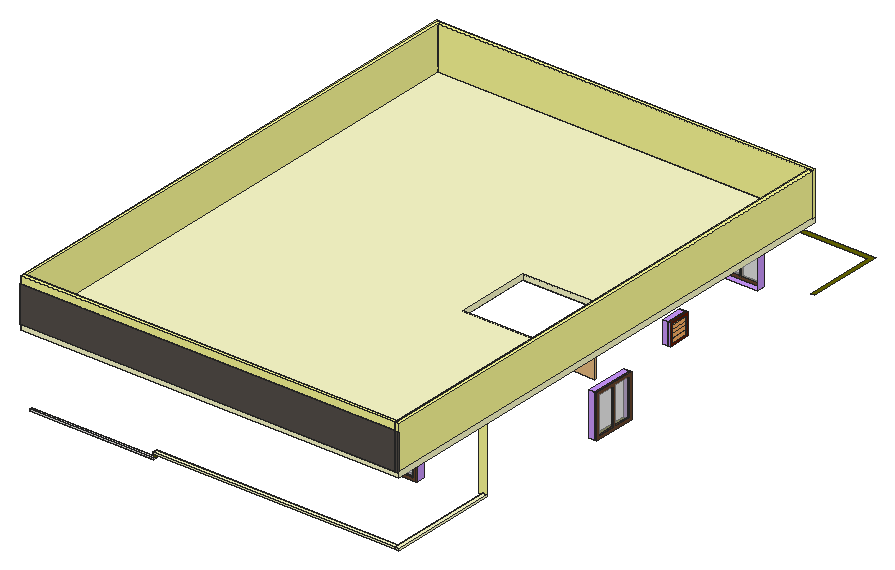
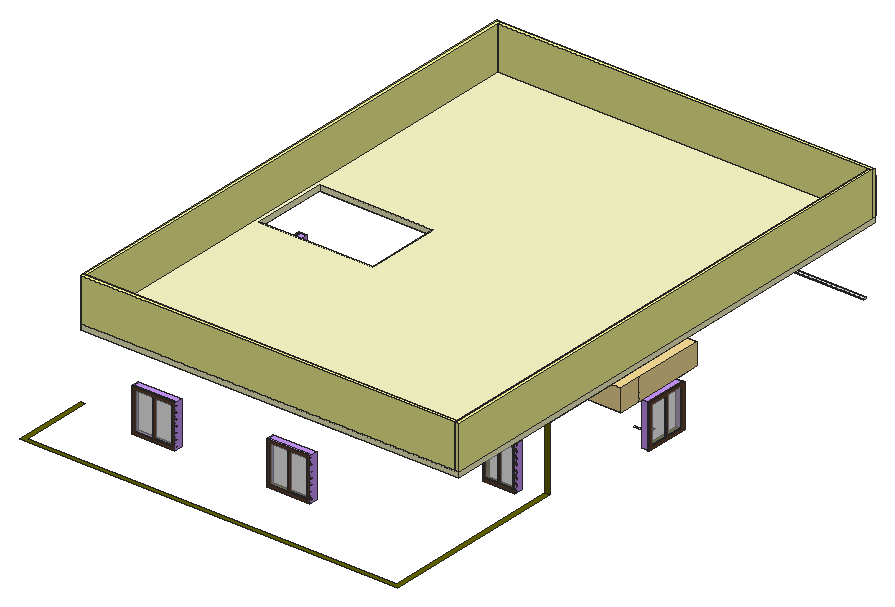
# SketchUp Ruby script. Lengths in inches.
U = 1.inch
M = Sketchup.active_model
def pt(a) = Geom::Point3d.new(a.map { |v| v * U })
def face(e, loops, mat)
  f = e.add_face(loops[0].map { |a| pt(a) })
  loops[1..].each { |l| e.add_face(l.map { |a| pt(a) }).erase! }
  f.material = f.back_material = mat if mat
  f
end
# faces: each face lists its corners as indices into pts; further lists are holes
def faces(e, pts, list, mat = nil) = list.each { |f| face(e, (f[0].is_a?(Array) ? f : [f]).map { |l| l.map { |i| pts[i] } }, mat) }
# xy, xz, yz: faces in a plane at the given z, y or x. An outline is a flat list of corners, or four numbers for a rectangle; further outlines are holes
def ring(l) = l.size == 4 ? [[l[0], l[1]], [l[2], l[1]], [l[2], l[3]], [l[0], l[3]]] : l.each_slice(2).to_a
def flat(e, list, mat, &to3) = list.each { |f| face(e, (f[0].is_a?(Array) ? f : [f]).map { |l| ring(l).map { |u, v| to3.(u, v) } }, mat) }
def xy(e, z, list, mat = nil) = flat(e, list, mat) { |x, y| [x, y, z] }
def xz(e, y, list, mat = nil) = flat(e, list, mat) { |x, z| [x, y, z] }
def yz(e, x, list, mat = nil) = flat(e, list, mat) { |y, z| [x, y, z] }
def lines(e, pts, list) = list.each { |a, b| e.add_line(pt(pts[a]), pt(pts[b])) }
# prism: a flat outline (further loops are holes) pulled along v
def prism(e, loops, v, mat = nil)
  f = face(e, loops, mat); d = Geom::Vector3d.new(v.map { |x| x * U })
  f.pushpull(f.normal.samedirection?(d) ? d.length : -d.length)
end
def box(e, o, s, mat = nil) = prism(e, [[o, [o[0] + s[0], o[1], o[2]], [o[0] + s[0], o[1] + s[1], o[2]], [o[0], o[1] + s[1], o[2]]]], [0, 0, s[2]], mat)
def at(x, y, z, deg = 0) = Geom::Transformation.translation(pt([x, y, z])) * Geom::Transformation.rotation(ORIGIN, Z_AXIS, deg.degrees)
def axes(o, x, y, z) = Geom::Transformation.new([*x, 0, *y, 0, *z, 0, *pt(o).to_a, 1])
def part(name) = M.definitions.add(name)
# library, detail: a bought-in or finely detailed component or shape, given as its bounding box
def library(name, o, s) = part(name).tap { |d| box(d.entities, o, s) }
def detail(e, o, s) = box(e.add_group.entities, o, s)
def put(e, d, t, mat = nil) = e.add_instance(d, t).tap { |i| i.material = mat if mat }
def group(e, t, mat = nil) = e.add_group.tap { |g| g.transformation = t; g.material = mat if mat }.entities
root = M.entities
M.materials.add("B08_Burnt_Sienna").color = [102, 25, 0]
M.materials.add("C03_Honey_Glow").color = [255, 178, 101]
M.materials.add("D02_Buttercup_Glow").color = [255, 229, 155]
M.materials.add("E01_Mint_Frost").color = [255, 255, 204]
M.materials.add("E02_Pale_Lime").color = [255, 255, 153]
M.materials.add("E08_Lime_Depth").color = [102, 102, 0]
M.materials.add("F06_Grassy_Shade").color = [102, 204, 0]
M.materials.add("G07_Jungle_Burst").color = [0, 153, 0]
M.materials.add("Glass_Mirror_01").color = [185, 185, 185]
M.materials["Glass_Mirror_01"].alpha = 0.91
M.materials.add("Glass_Mirror_2").color = [185, 185, 185]
M.materials["Glass_Mirror_2"].alpha = 0.8
M.materials.add("Glass_Mirror_3").color = [185, 185, 185]
M.materials["Glass_Mirror_3"].alpha = 0.65
M.materials.add("Glass_Mirror_4").color = [185, 185, 185]
M.materials["Glass_Mirror_4"].alpha = 0.68
M.materials.add("H06_Ocean_Depth").color = [0, 204, 204]
M.materials.add("H08_Emerald_Abyss").color = [0, 102, 102]
M.materials.add("I03_Bluebell_Mist").color = [101, 101, 255]
M.materials.add("I08_Inkstorm").color = [0, 0, 102]
M.materials.add("J02_Lavender_Veil").color = [204, 153, 255]
M.materials.add("J03_Orchid_Glow").color = [178, 101, 255]
M.materials.add("K02_Rosy_Glow").color = [255, 153, 255]
M.materials.add("M07_Charcoal_Gleam").color = [58, 58, 58]
M.materials.add("M09_Shadow_Night").color = [0, 0, 0]
M.materials.add("Metal_06_1K").color = [238, 236, 231]
M.materials.add("Roofing_01_1K").color = [84, 79, 73]
M.materials.add("Wood_Veneer_15_1K").color = [103, 69, 45]
c1 = part("Group\#57")
xy(c1.entities,0,[[0,-2,48,0]],"Wood_Veneer_15_1K")
xy(c1.entities,3,[[3,-2,23,0],[25,-2,45,0]],"Wood_Veneer_15_1K")
xy(c1.entities,45,[[3,-2,23,0],[25,-2,45,0]],"Wood_Veneer_15_1K")
xy(c1.entities,48,[[0,-2,48,0]],"Wood_Veneer_15_1K")
xz(c1.entities,-2,[[[0,0,48,48],[25,3,45,45],[3,3,23,45]]],"Wood_Veneer_15_1K")
xz(c1.entities,0,[[3,3,23,45],[25,3,45,45]],"Glass_Mirror_4")
xz(c1.entities,0,[[[0,0,48,48],[25,3,45,45],[3,3,23,45]]],"Wood_Veneer_15_1K")
yz(c1.entities,0,[[-2,0,0,48]],"Wood_Veneer_15_1K")
yz(c1.entities,3,[[-2,3,0,45]],"Wood_Veneer_15_1K")
yz(c1.entities,23,[[-2,3,0,45]],"Wood_Veneer_15_1K")
yz(c1.entities,25,[[-2,3,0,45]],"Wood_Veneer_15_1K")
yz(c1.entities,45,[[-2,3,0,45]],"Wood_Veneer_15_1K")
yz(c1.entities,48,[[-2,0,0,48]],"Wood_Veneer_15_1K")
c2 = library("Group\#24",[0,0,0],[4.375,4.375,0.1875])
c3 = part("Group\#8")
g1 = group(c3.entities,at(0.75,15.42,1.1875),"M07_Charcoal_Gleam")
prism(g1,[[[1.25,5.68,0],[1.25,0.93,0],[0.46,0.6,0],[0.3125,0.54,0],[0.18,0.44,0],[0.08,0.3125,0],[0.02,0.16,0],[0,0,0],[0,6.6875,0],[0.02,6.53,0],[0.08,6.375,0],[0.18,6.25,0],[0.3125,6.15,0],[0.46,6.08,0],[0.625,6.0625,0]]],[0,0,3.25])
g2 = group(c3.entities,at(0,11.83,0))
box(g2,[0,0,0],[2.8125,14.875,1.1875],"M07_Charcoal_Gleam")
g3 = group(c3.entities,at(2,0,4.4375))
xy(g3,0,[[-1,0,0,37.44]],"M07_Charcoal_Gleam")
xy(g3,21.9,[[-1,0,0,37.44]],"M07_Charcoal_Gleam")
xz(g3,0,[[-1,0,0,21.9]],"M07_Charcoal_Gleam")
xz(g3,37.44,[[-1,0,0,21.9]],"M07_Charcoal_Gleam")
yz(g3,-1,[[1.62,1.96,35.68,20.27]],"Glass_Mirror_01")
yz(g3,-1,[[[0,0,37.44,21.9],[1.62,1.96,35.68,20.27]]],"M07_Charcoal_Gleam")
yz(g3,0,[[[0,0,37.44,21.9],[1.62,1.96,35.68,20.27]]],"M07_Charcoal_Gleam")
p = [[0,35.68,20.27],[-1,35.68,20.27],[0,1.62,20.27],[-1,1.62,20.27],[0,35.68,1.96],[-1,35.68,1.96],
  [0,1.62,1.96],[-1,1.62,1.96]]
lines(g3,p,[[0,1],[2,3],[4,5],[6,7]])
c4 = part("Group\#56")
xy(c4.entities,0,[[0,0,2,48]],"Wood_Veneer_15_1K")
xy(c4.entities,3,[[0,3,2,23],[0,25,2,45]],"Wood_Veneer_15_1K")
xy(c4.entities,45.04,[[0,3,2,23],[0,25,2,45]],"Wood_Veneer_15_1K")
xy(c4.entities,48.04,[[0,0,2,48]],"Wood_Veneer_15_1K")
xz(c4.entities,0,[[0,0,2,48.04]],"Wood_Veneer_15_1K")
xz(c4.entities,3,[[0,3,2,23.02],[0,23.02,2,25.02],[0,25.02,2,45.04]],"Wood_Veneer_15_1K")
xz(c4.entities,23,[[0,3,2,23.02],[0,23.02,2,25.02],[0,25.02,2,45.04]],"Wood_Veneer_15_1K")
xz(c4.entities,25,[[0,3,2,23.02],[0,23.02,2,25.02],[0,25.02,2,45.04]],"Wood_Veneer_15_1K")
xz(c4.entities,45,[[0,3,2,23.02],[0,23.02,2,25.02],[0,25.02,2,45.04]],"Wood_Veneer_15_1K")
xz(c4.entities,48,[[0,0,2,48.04]],"Wood_Veneer_15_1K")
yz(c4.entities,0,[[3,3,23,45.04],[25,3,45,45.04]],"Glass_Mirror_3")
yz(c4.entities,0,[[[0,0,48,48.04],[3,3,23,45.04],[25,3,45,45.04]]],"Wood_Veneer_15_1K")
yz(c4.entities,2,[[[0,0,48,48.04],[3,3,23,45.04],[25,3,45,45.04]]],"Wood_Veneer_15_1K")
c5 = library("Group\#23",[0,0,0],[35.8125,17,3.54])
c6 = part("Group\#44")
detail(c6.entities,[0,0,0],[24,1.25,24])
c7 = part("Group\#66")
xy(c7.entities,0,[[0,0,27.25,1]],"M09_Shadow_Night")
xy(c7.entities,1.6,[[1.6,0.125,25.65,1]])
xy(c7.entities,1.6,[[1.6,0,25.65,0.125]],"M09_Shadow_Night")
xy(c7.entities,18.71,[[1.6,0.125,25.65,1]])
xy(c7.entities,18.71,[[1.6,0,25.65,0.125]],"M09_Shadow_Night")
xy(c7.entities,20.3125,[[0,0,27.25,1]],"M09_Shadow_Night")
xz(c7.entities,0,[[[0,0,27.25,20.3125],[1.6,1.6,25.65,18.71]]],"M09_Shadow_Night")
xz(c7.entities,0.125,[[[25.65,15.53,11.53,18.71,25.65,18.71],[25.29,15.97,25.29,18.36,14.71,18.36]]],"F06_Grassy_Shade")
xz(c7.entities,0.125,[[25.29,15.97,14.71,18.36,25.29,18.36]],"G07_Jungle_Burst")
xz(c7.entities,0.125,[[[10.47,1.6,12.94,7.09,17,16.09,23.34,1.6],[11.43,2.22,22.39,2.22,16.99,14.5625,13.51,6.83]]],"H06_Ocean_Depth")
xz(c7.entities,0.125,[[11.43,2.22,13.51,6.83,16.99,14.5625,22.39,2.22]],"H08_Emerald_Abyss")
xz(c7.entities,0.125,[[[1.6,1.6,1.6,15.53,12.94,7.09,10.47,1.6],[2.22,2.22,10.07,2.22,12.18,6.89,2.22,14.29]]],"I03_Bluebell_Mist")
xz(c7.entities,0.125,[[2.22,2.22,2.22,14.29,12.18,6.89,10.07,2.22]],"I08_Inkstorm")
xz(c7.entities,0.125,[[23.64,2.06,17.1,16.99,25.19,15.16,25.19,2.06],[12.76,7.79,2.06,15.75,2.06,18.25,11.48,18.25,16.92,17.03]],"J03_Orchid_Glow")
xz(c7.entities,0.125,[[[23.34,1.6,17,16.09,12.94,7.09,1.6,15.53,1.6,18.71,11.53,18.71,25.65,15.53,25.65,1.6],[12.76,7.79,16.92,17.03,11.48,18.25,2.06,18.25,2.06,15.75],[23.64,2.06,25.19,2.06,25.19,15.16,17.1,16.99]]],"K02_Rosy_Glow")
xz(c7.entities,1,[[[0,0,27.25,20.3125],[1.6,1.6,25.65,18.71]]],"M09_Shadow_Night")
yz(c7.entities,0,[[0,0,1,20.3125]],"M09_Shadow_Night")
yz(c7.entities,1.6,[[0.125,1.6,1,18.71]])
yz(c7.entities,1.6,[[0,1.6,0.125,18.71]],"M09_Shadow_Night")
yz(c7.entities,25.65,[[0.125,1.6,1,18.71]])
yz(c7.entities,25.65,[[0,1.6,0.125,18.71]],"M09_Shadow_Night")
yz(c7.entities,27.25,[[0,0,1,20.3125]],"M09_Shadow_Night")
c8 = part("Group\#37")
xy(c8.entities,0,[[0,0,52.33,16.76],[94.85,0,137.375,16.76],[0,16.76,0,104.9375,66.09,104.9375,66.09,88.6875,18.42,88.6875,18.42,16.76]],"D02_Buttercup_Glow")
xy(c8.entities,0,[[52.33,0,94.85,16.76]],"M07_Charcoal_Gleam")
xy(c8.entities,24.5625,[[0,0,52.33,0,52.33,16.76,18.42,16.76,18.42,88.6875,66.09,88.6875,66.09,104.9375,0,104.9375],[94.85,0,137.375,16.76]],"D02_Buttercup_Glow")
xz(c8.entities,0,[[0,0,52.33,24.5625],[94.85,0,137.375,24.5625]],"D02_Buttercup_Glow")
xz(c8.entities,0,[[52.33,0,94.85,2.0625]],"M07_Charcoal_Gleam")
xz(c8.entities,16.76,[[[18.42,0,52.33,24.5625],[20.03,1.61,50.72,22.95]],[[94.85,0,116.11,24.5625],[96.47,1.61,114.5,22.95]],[[116.11,0,137.375,24.5625],[117.8125,1.7,135.68,22.87]]],"D02_Buttercup_Glow")
xz(c8.entities,16.76,[[20.03,1.61,50.72,22.95],[96.47,1.61,114.5,22.95],[117.8125,1.7,135.68,22.87]],"Glass_Mirror_2")
xz(c8.entities,16.76,[[52.33,0,94.85,2.0625]],"M07_Charcoal_Gleam")
xz(c8.entities,88.6875,[[[18.42,0,42.25,24.5625],[20.03,1.61,40.64,22.95]],[[42.25,0,66.09,24.5625],[43.87,1.61,64.48,22.95]]],"D02_Buttercup_Glow")
xz(c8.entities,88.6875,[[20.03,1.61,40.64,22.95],[43.87,1.61,64.48,22.95]],"Glass_Mirror_2")
xz(c8.entities,104.9375,[[0,0,66.09,24.5625]],"D02_Buttercup_Glow")
yz(c8.entities,0,[[0,0,80.9375,24.5625],[80.9375,0,104.9375,24.5625]],"D02_Buttercup_Glow")
yz(c8.entities,18.42,[[[16.76,0,40.76,24.5625],[18.37,1.61,39.15,22.95]],[[40.76,0,64.76,24.5625],[42.37,1.61,63.15,22.95]],[[64.76,0,88.6875,24.5625],[66.37,1.61,87.08,22.95]]],"D02_Buttercup_Glow")
yz(c8.entities,18.42,[[18.37,1.61,39.15,22.95],[42.37,1.61,63.15,22.95],[66.37,1.61,87.08,22.95]],"Glass_Mirror_2")
yz(c8.entities,52.33,[[0,2.0625,16.76,24.5625]],"D02_Buttercup_Glow")
yz(c8.entities,52.33,[[0,0,16.76,2.0625]],"M07_Charcoal_Gleam")
yz(c8.entities,66.09,[[88.6875,0,104.9375,24.5625]],"D02_Buttercup_Glow")
yz(c8.entities,94.85,[[0,2.0625,16.76,24.5625]],"D02_Buttercup_Glow")
yz(c8.entities,94.85,[[0,0,16.76,2.0625]],"M07_Charcoal_Gleam")
yz(c8.entities,137.375,[[0,0,16.76,24.5625]],"D02_Buttercup_Glow")
g4 = group(c8.entities,at(67.95,4.33,2.0625))
xy(g4,0,[[[-15.61,-4.33,26.91,12.43],[0,0,13.8125,6.75]],[0,0,13.8125,6.75]],"M07_Charcoal_Gleam")
xy(g4,6.25,[[0,0,13.8125,6.75]],"M07_Charcoal_Gleam")
xy(g4,22.5,[[0,0,13.8125,6.75]],"M07_Charcoal_Gleam")
xz(g4,0,[[0,0,13.8125,6.25],[0,6.25,13.8125,22.5]],"M07_Charcoal_Gleam")
xz(g4,6.75,[[0,0,13.8125,6.25],[0,6.25,13.8125,22.5]],"M07_Charcoal_Gleam")
yz(g4,0,[[0,0,6.75,6.25],[0,6.25,6.75,22.5]],"M07_Charcoal_Gleam")
yz(g4,13.8125,[[0,0,6.75,6.25],[0,6.25,6.75,22.5]],"M07_Charcoal_Gleam")
p = [[-15.61,-4.33,0],[0,0,6.25],[0,6.75,6.25],[-15.61,12.43,0],[26.91,-4.33,0],[13.8125,0,6.25],
  [26.91,12.43,0],[13.8125,6.75,6.25]]
faces(g4,p,[[0,1,2,3],[4,5,1,0],[4,6,7,5],[3,2,7,6]],"M07_Charcoal_Gleam")
c9 = part("Group\#58")
xy(c9.entities,0,[[0,0,2.5,24]],"B08_Burnt_Sienna")
xy(c9.entities,1.73,[[1,1.73,2.5,22.27]],"B08_Burnt_Sienna")
xy(c9.entities,1.73,[[0,1.73,1,22.27]],"C03_Honey_Glow")
xy(c9.entities,6.06,[[0,1.73,1,22.27]],"C03_Honey_Glow")
xy(c9.entities,6.54,[[0,1.73,1,22.27]],"C03_Honey_Glow")
xy(c9.entities,10.31,[[0,1.73,1,22.27]],"C03_Honey_Glow")
xy(c9.entities,10.84,[[0,1.73,1,22.27]],"C03_Honey_Glow")
xy(c9.entities,14.12,[[0,1.73,1,22.27]],"C03_Honey_Glow")
xy(c9.entities,14.57,[[0,1.73,1,22.27]],"C03_Honey_Glow")
xy(c9.entities,18.12,[[0,1.73,1,22.27]],"C03_Honey_Glow")
xy(c9.entities,18.66,[[0,1.73,1,22.27]],"C03_Honey_Glow")
xy(c9.entities,22.27,[[1,1.73,2.5,22.27]],"B08_Burnt_Sienna")
xy(c9.entities,22.27,[[0,1.73,1,22.27]],"C03_Honey_Glow")
xy(c9.entities,24,[[0,0,2.5,24]],"B08_Burnt_Sienna")
xz(c9.entities,0,[[0,0,2.5,24]],"B08_Burnt_Sienna")
xz(c9.entities,1.73,[[0,18.12,1,18.66]])
xz(c9.entities,1.73,[[1,1.73,1,6.06,0,6.06,0,6.54,1,6.54,1,10.31,0,10.31,0,10.84,1,10.84,1,14.12,0,14.12,0,14.57,1,14.57,1,22.27,2.5,22.27,2.5,1.73]],"B08_Burnt_Sienna")
xz(c9.entities,1.73,[[0,1.73,1,6.06],[0,6.54,1,10.31],[0,10.84,1,14.12],[0,14.57,1,18.12],[0,18.66,1,22.27]],"C03_Honey_Glow")
xz(c9.entities,22.27,[[0,18.12,1,18.66]])
xz(c9.entities,22.27,[[1,1.73,2.5,1.73,2.5,22.27,1,22.27,1,14.57,0,14.57,0,14.12,1,14.12,1,10.84,0,10.84,0,10.31,1,10.31,1,6.54,0,6.54,0,6.06,1,6.06]],"B08_Burnt_Sienna")
xz(c9.entities,22.27,[[0,1.73,1,6.06],[0,6.54,1,10.31],[0,10.84,1,14.12],[0,14.57,1,18.12],[0,18.66,1,22.27]],"C03_Honey_Glow")
xz(c9.entities,24,[[0,0,2.5,24]],"B08_Burnt_Sienna")
yz(c9.entities,0,[[[0,0,24,24],[1.73,1.73,22.27,22.27]]],"B08_Burnt_Sienna")
yz(c9.entities,0,[[1.73,1.73,22.27,6.06],[1.73,6.54,22.27,10.31],[1.73,10.84,22.27,14.12],[1.73,14.57,22.27,18.12],[1.73,18.66,22.27,22.27]],"C03_Honey_Glow")
yz(c9.entities,1,[[1.73,1.73,22.27,6.06],[1.73,6.54,22.27,10.31],[1.73,10.84,22.27,14.12],[1.73,14.57,22.27,18.12],[1.73,18.66,22.27,22.27]],"C03_Honey_Glow")
yz(c9.entities,2.5,[[[0,0,24,24],[1.73,1.73,22.27,22.27]]],"B08_Burnt_Sienna")
box(root,[1722.42,1900.1875,273.24],[65.69,12,20.76],"E08_Lime_Depth")
xy(root,204,[[1567.04,2005.11,1576.04,2053.11]],"E08_Lime_Depth")
xy(root,210,[[1978.04,2015.58,1987.04,2063.58],[1605.14,2183.58,1641.14,2192.58],[1732.04,2309.58,1780.04,2318.58]],"E08_Lime_Depth")
xy(root,210,[[1862.07,1862.58,1910.07,1871.58],[1882.04,2309.58,1930.04,2318.58]],"J02_Lavender_Veil")
xy(root,211,[[1579.51,2036.36,1597.51,2036.99]],"Metal_06_1K")
xy(root,216.0625,[[1576.04,1741.67,1714.42,1745.11]],"Metal_06_1K")
xy(root,217.5625,[[1576.04,1741.67,1714.42,1745.11]],"Metal_06_1K")
xy(root,222,[[1714.42,1740.42,1982.36,1745.11],[1982.36,1740.42,1987.04,1862.58]],"E01_Mint_Frost")
xy(root,222,[[1567.04,2192.58,1571.73,2192.58,1571.73,2397.95,1982.36,2397.95,1982.36,2318.58,1987.04,2318.58,1987.04,2402.64,1567.04,2402.64]],"E08_Lime_Depth")
xy(root,224,[[1714.42,1740.42,1982.36,1745.11],[1982.36,1740.42,1987.04,1862.58]],"E01_Mint_Frost")
xy(root,246,[[1713.42,1916.04,1722.42,1940.04]],"J02_Lavender_Veil")
xy(root,252,[[1567.04,2005.11,1576.04,2053.11]],"J02_Lavender_Veil")
xy(root,258,[[1862.07,1862.58,1910.07,1871.58],[1788.11,1951.47,1794.11,1985.89],[1798.45,1991.58,1840.09,1997.58],[1644.54,2081.58,1675.875,2087.58],[1888.04,2137.61,1894.04,2167.61],
  [1788.97,2171.58,1824.97,2177.58],[1837.82,2171.58,1873.82,2177.58],[1605.14,2183.58,1675.875,2192.58],[1732.04,2309.58,1780.04,2318.58],[1882.04,2309.58,1930.04,2318.58]],"J02_Lavender_Veil")
xy(root,258.0625,[[1641.14,2183.58,1644.54,2192.58]],"E08_Lime_Depth")
xy(root,258.9375,[[1978.04,2117.58,1987.04,2141.58]],"E08_Lime_Depth")
xy(root,282.9375,[[1978.04,2117.58,1987.04,2141.58]],"J02_Lavender_Veil")
xy(root,294,[[1567.04,1740.42,1576.04,1967.64]],"E08_Lime_Depth")
xy(root,294,[[[1713.42,1862.58,1722.42,1862.58,1722.42,2000.64,1713.42,2000.64,1713.42,1976.64,1576.04,1976.64,1576.04,2081.58,1684.04,2081.58,1684.04,2171.58,1888.04,2171.58,1888.04,2081.58,1978.04,2081.58,1978.04,1997.58,1788.11,1997.58,1788.11,1862.58,1987.04,1862.58,1987.04,2318.58,1678.04,2318.58,1678.04,2192.58,1567.04,2192.58,1567.04,1967.64,1713.42,1967.64],[1794.11,1871.58,1978.04,1991.58],[1684.04,2177.58,1828.04,2309.58],[1834.04,2177.58,1978.04,2309.58],[1576.04,2087.58,1678.04,2183.58],[1894.04,2087.58,1978.04,2171.58]]],"J02_Lavender_Veil")
xz(root,1740.42,[[1714.42,222,1982.36,224],[1982.36,222,1987.04,224]],"E01_Mint_Frost")
xz(root,1741.67,[[1576.04,216.0625,1714.42,217.5625]],"Metal_06_1K")
xz(root,1745.11,[[1714.42,222,1982.36,224]],"E01_Mint_Frost")
xz(root,1745.11,[[1576.04,216.0625,1714.42,217.5625]],"Metal_06_1K")
xz(root,1862.58,[[1982.36,222,1987.04,224]],"E01_Mint_Frost")
xz(root,1862.58,[[1978.04,222,1982.36,222,1982.36,224,1987.04,224,1987.04,294,1978.04,294]],"E02_Pale_Lime")
xz(root,1940.04,[[1713.42,210,1722.42,246]],"J02_Lavender_Veil")
xz(root,2005.11,[[1567.04,204,1576.04,252]],"J02_Lavender_Veil")
xz(root,2015.58,[[1978.04,210,1978.04,258,1987.04,258.04,1987.04,210]],"J02_Lavender_Veil")
xz(root,2053.11,[[1567.04,204,1576.04,252]],"J02_Lavender_Veil")
xz(root,2063.58,[[1978.04,210,1987.04,210,1987.04,258.04,1978.04,258]],"J02_Lavender_Veil")
xz(root,2117.58,[[1978.04,258.9375,1987.04,282.9375]],"J02_Lavender_Veil")
xz(root,2141.58,[[1978.04,258.9375,1987.04,282.9375]],"J02_Lavender_Veil")
xz(root,2183.58,[[1641.14,258,1644.54,258.0625]],"J02_Lavender_Veil")
xz(root,2192.58,[[1567.04,222,1571.73,294]],"E08_Lime_Depth")
xz(root,2192.58,[[1641.14,258,1644.54,258.0625]],"J02_Lavender_Veil")
yz(root,1576.04,[[1741.67,216.0625,1745.11,217.5625]],"Metal_06_1K")
yz(root,1605.14,[[2183.58,210,2192.58,258]],"J02_Lavender_Veil")
yz(root,1641.14,[[2183.58,210,2192.58,258.0625]],"E08_Lime_Depth")
yz(root,1714.42,[[1740.42,222,1741.67,224],[1741.67,222,1745.11,224]],"E01_Mint_Frost")
yz(root,1714.42,[[1741.67,217.5625,1745.11,222]],"E08_Lime_Depth")
yz(root,1714.42,[[1741.67,216.0625,1745.11,217.5625]],"Metal_06_1K")
yz(root,1732.04,[[2309.58,210,2318.58,258]],"J02_Lavender_Veil")
yz(root,1780.04,[[2309.58,210,2318.58,258]],"J02_Lavender_Veil")
yz(root,1862.07,[[1862.58,210,1871.58,258]],"J02_Lavender_Veil")
yz(root,1882.04,[[2309.58,210,2318.58,258]],"J02_Lavender_Veil")
yz(root,1910.07,[[1862.58,210,1871.58,258]],"J02_Lavender_Veil")
yz(root,1930.04,[[2309.58,210,2318.58,258]],"J02_Lavender_Veil")
yz(root,1982.36,[[1740.42,222,1745.11,224],[1745.11,222,1862.58,224]],"E01_Mint_Frost")
yz(root,1987.04,[[1740.42,222,1862.58,224]],"E01_Mint_Frost")
p = [[1987.04,2015.58,258.04],[1978.04,2015.58,258],[1978.04,2063.58,258],[1987.04,2063.58,258.04],[1675.875,2087.58,258],[1675.875,2081.58,258]]
faces(root,p,[[0,1,2,3]],"J02_Lavender_Veil")
lines(root,p,[[4,5]])
put(root,c1,at(1569.04,2053.11,204,-90),"E02_Pale_Lime")
put(root,c2,at(1587.56,2020.89,205.1875),"E08_Lime_Depth")
put(root,c1,axes([1641.14,2190.58,210],[-0.75,0,0],[0,-1,0],[0,0,1]),"E02_Pale_Lime")
put(root,c3,at(1807.5,1896.67,210),"E08_Lime_Depth")
put(root,c4,at(1985.04,2015.58,210),"E02_Pale_Lime")
put(root,c1,at(1862.07,1862.58,210),"E02_Pale_Lime")
put(root,c1,at(1930.04,2316.58,210,180),"E02_Pale_Lime")
put(root,c1,at(1780.04,2316.58,210,180),"E02_Pale_Lime")
put(root,c5,at(1630.1,1980.73,211),"E08_Lime_Depth")
put(root,c6,at(1901.77,2089.5,216.93),"E08_Lime_Depth")
put(root,c7,at(1827.5,1871.58,237.49),"E02_Pale_Lime")
put(root,c8,at(1576.04,1976.64,252),"E08_Lime_Depth")
put(root,c9,at(1984.54,2117.58,258.9375),"E02_Pale_Lime")
g5 = group(root,at(1567.04,1740.42,294),"E08_Lime_Depth")
prism(g5,[[[420,0,0],[0,0,0],[0,578.15,0],[420,578.15,0]],[[285,257.15,0],[411,257.15,0],[411,341.15,0],[285,341.15,0]]],[0,0,6],"E01_Mint_Frost")
g6 = group(root,at(1567.04,1740.42,300),"E02_Pale_Lime")
xy(g6,0,[[0,0,416,4],[416,0,420,574.15],[0,4,4,578.15],[4,574.15,420,578.15]])
xy(g6,48,[[0,0,416,4],[416,0,420,574.15],[0,4,4,578.15],[4,574.15,420,578.15]])
xz(g6,0,[[416,0,420,39.89],[0,39.89,416,48],[416,39.89,420,48]])
xz(g6,4,[[4,0,416,48]])
xz(g6,574.15,[[4,0,416,48],[416,0,420,48]])
xz(g6,578.15,[[0,0,4,48],[4,0,420,48]])
yz(g6,0,[[0,0,4,48],[4,0,578.15,48]])
yz(g6,4,[[4,0,574.15,48],[574.15,0,578.15,48]])
yz(g6,416,[[0,0,4,48],[4,0,574.15,48]])
yz(g6,420,[[0,0,574.15,48],[574.15,0,578.15,48]])
g7 = group(g6,at(0,0,0),"Roofing_01_1K")
box(g7,[0,-1,0],[420,1,39.89])
